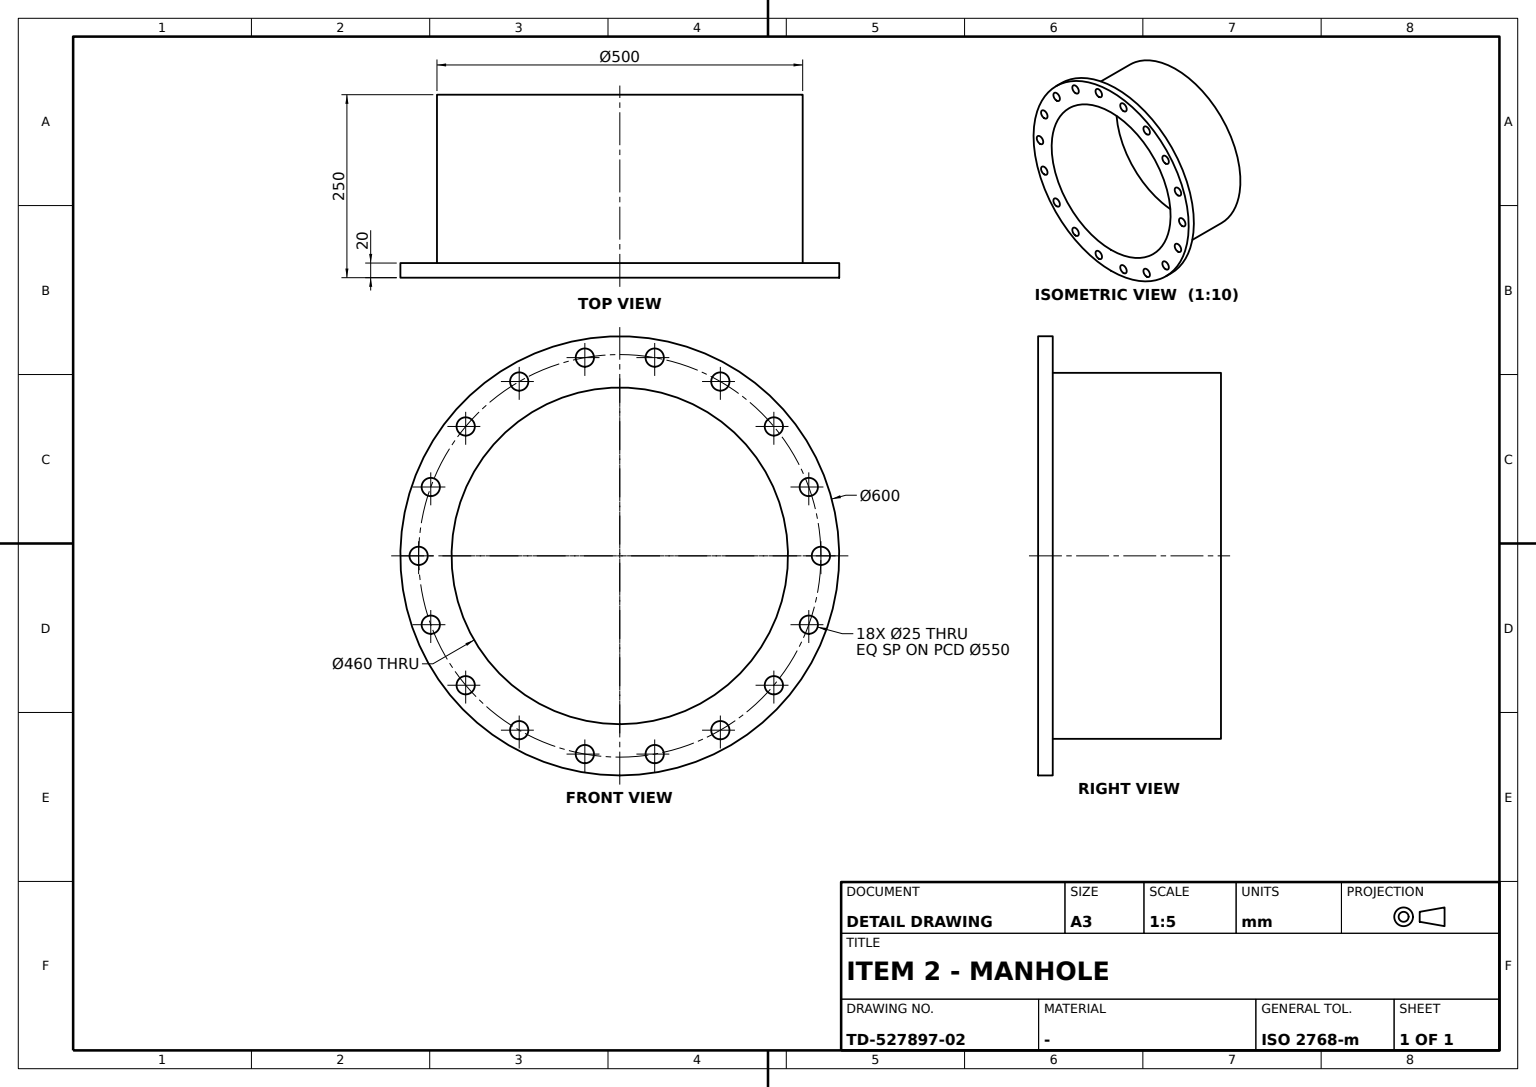
ISO-10303-21;
HEADER;
FILE_DESCRIPTION((''),'2;1');
FILE_NAME('','',(''),(''),'','','');
FILE_SCHEMA(('AUTOMOTIVE_DESIGN'));
ENDSEC;
DATA;
#1=APPLICATION_CONTEXT('');
#2=PRODUCT_CONTEXT('',#1,'mechanical');
#3=PRODUCT('','','',(#2));
#4=PRODUCT_DEFINITION_FORMATION('','',#3);
#5=PRODUCT_DEFINITION_CONTEXT('',#1,'design');
#6=PRODUCT_DEFINITION('','',#4,#5);
#7=PRODUCT_DEFINITION_SHAPE('','',#6);
#8=(LENGTH_UNIT()NAMED_UNIT(*)SI_UNIT(.MILLI.,.METRE.));
#9=(NAMED_UNIT(*)PLANE_ANGLE_UNIT()SI_UNIT($,.RADIAN.));
#10=(NAMED_UNIT(*)SI_UNIT($,.STERADIAN.)SOLID_ANGLE_UNIT());
#11=UNCERTAINTY_MEASURE_WITH_UNIT(LENGTH_MEASURE(0.005),#8,'distance_accuracy_value','');
#12=(GEOMETRIC_REPRESENTATION_CONTEXT(3)GLOBAL_UNCERTAINTY_ASSIGNED_CONTEXT((#11))GLOBAL_UNIT_ASSIGNED_CONTEXT((#8,#9,#10))REPRESENTATION_CONTEXT('',''));
#13=CARTESIAN_POINT('',(250.656986,-137.5,2750.));
#14=VERTEX_POINT('',#13);
#15=CARTESIAN_POINT('',(238.156986,-137.5,2750.));
#16=DIRECTION('',(0.,0.,1.));
#17=DIRECTION('',(1.,0.,0.));
#18=AXIS2_PLACEMENT_3D('',#15,#16,#17);
#19=CIRCLE('',#18,12.5);
#20=EDGE_CURVE('',#14,#14,#19,.T.);
#21=ORIENTED_EDGE('',*,*,#20,.T.);
#22=EDGE_LOOP('',(#21));
#23=FACE_BOUND('',#22,.T.);
#24=CARTESIAN_POINT('',(250.656986,-137.5,2730.));
#25=VERTEX_POINT('',#24);
#26=CARTESIAN_POINT('',(238.156986,-137.5,2730.));
#27=AXIS2_PLACEMENT_3D('',#26,#16,#17);
#28=CIRCLE('',#27,12.5);
#29=EDGE_CURVE('',#25,#25,#28,.T.);
#30=ORIENTED_EDGE('',*,*,#29,.F.);
#31=EDGE_LOOP('',(#30));
#32=FACE_BOUND('',#31,.T.);
#33=CARTESIAN_POINT('',(238.156986,-137.5,2740.));
#34=AXIS2_PLACEMENT_3D('',#33,#16,#17);
#35=CYLINDRICAL_SURFACE('',#34,12.5);
#36=ADVANCED_FACE('',(#23,#32),#35,.F.);
#37=CARTESIAN_POINT('',(-164.266593,-210.662222,2750.));
#38=VERTEX_POINT('',#37);
#39=CARTESIAN_POINT('',(-176.766593,-210.662222,2750.));
#40=AXIS2_PLACEMENT_3D('',#39,#16,#17);
#41=CIRCLE('',#40,12.5);
#42=EDGE_CURVE('',#38,#38,#41,.T.);
#43=ORIENTED_EDGE('',*,*,#42,.T.);
#44=EDGE_LOOP('',(#43));
#45=FACE_BOUND('',#44,.T.);
#46=CARTESIAN_POINT('',(-164.266593,-210.662222,2730.));
#47=VERTEX_POINT('',#46);
#48=CARTESIAN_POINT('',(-176.766593,-210.662222,2730.));
#49=AXIS2_PLACEMENT_3D('',#48,#16,#17);
#50=CIRCLE('',#49,12.5);
#51=EDGE_CURVE('',#47,#47,#50,.T.);
#52=ORIENTED_EDGE('',*,*,#51,.F.);
#53=EDGE_LOOP('',(#52));
#54=FACE_BOUND('',#53,.T.);
#55=CARTESIAN_POINT('',(-176.766593,-210.662222,2740.));
#56=AXIS2_PLACEMENT_3D('',#55,#16,#17);
#57=CYLINDRICAL_SURFACE('',#56,12.5);
#58=ADVANCED_FACE('',(#45,#54),#57,.F.);
#59=CARTESIAN_POINT('',(-81.555539,258.415471,2730.));
#60=VERTEX_POINT('',#59);
#61=CARTESIAN_POINT('',(-94.055539,258.415471,2730.));
#62=AXIS2_PLACEMENT_3D('',#61,#16,#17);
#63=CIRCLE('',#62,12.5);
#64=EDGE_CURVE('',#60,#60,#63,.T.);
#65=ORIENTED_EDGE('',*,*,#64,.F.);
#66=EDGE_LOOP('',(#65));
#67=FACE_BOUND('',#66,.T.);
#68=CARTESIAN_POINT('',(-81.555539,258.415471,2750.));
#69=VERTEX_POINT('',#68);
#70=CARTESIAN_POINT('',(-94.055539,258.415471,2750.));
#71=AXIS2_PLACEMENT_3D('',#70,#16,#17);
#72=CIRCLE('',#71,12.5);
#73=EDGE_CURVE('',#69,#69,#72,.T.);
#74=ORIENTED_EDGE('',*,*,#73,.T.);
#75=EDGE_LOOP('',(#74));
#76=FACE_BOUND('',#75,.T.);
#77=CARTESIAN_POINT('',(-94.055539,258.415471,2740.));
#78=AXIS2_PLACEMENT_3D('',#77,#16,#17);
#79=CYLINDRICAL_SURFACE('',#78,12.5);
#80=ADVANCED_FACE('',(#67,#76),#79,.F.);
#81=CARTESIAN_POINT('',(230.,0.,2750.));
#82=VERTEX_POINT('',#81);
#83=CARTESIAN_POINT('',(0.,0.,2750.));
#84=AXIS2_PLACEMENT_3D('',#83,#16,#17);
#85=CIRCLE('',#84,230.);
#86=EDGE_CURVE('',#82,#82,#85,.T.);
#87=ORIENTED_EDGE('',*,*,#86,.T.);
#88=EDGE_LOOP('',(#87));
#89=FACE_BOUND('',#88,.T.);
#90=CARTESIAN_POINT('',(230.,0.,2500.));
#91=VERTEX_POINT('',#90);
#92=CARTESIAN_POINT('',(0.,0.,2500.));
#93=AXIS2_PLACEMENT_3D('',#92,#16,#17);
#94=CIRCLE('',#93,230.);
#95=EDGE_CURVE('',#91,#91,#94,.T.);
#96=ORIENTED_EDGE('',*,*,#95,.F.);
#97=EDGE_LOOP('',(#96));
#98=FACE_BOUND('',#97,.T.);
#99=CARTESIAN_POINT('',(0.,0.,2625.));
#100=AXIS2_PLACEMENT_3D('',#99,#16,#17);
#101=CYLINDRICAL_SURFACE('',#100,230.);
#102=ADVANCED_FACE('',(#89,#98),#101,.F.);
#103=CARTESIAN_POINT('',(-225.656986,137.5,2730.));
#104=VERTEX_POINT('',#103);
#105=CARTESIAN_POINT('',(-238.156986,137.5,2730.));
#106=AXIS2_PLACEMENT_3D('',#105,#16,#17);
#107=CIRCLE('',#106,12.5);
#108=EDGE_CURVE('',#104,#104,#107,.T.);
#109=ORIENTED_EDGE('',*,*,#108,.F.);
#110=EDGE_LOOP('',(#109));
#111=FACE_BOUND('',#110,.T.);
#112=CARTESIAN_POINT('',(-225.656986,137.5,2750.));
#113=VERTEX_POINT('',#112);
#114=CARTESIAN_POINT('',(-238.156986,137.5,2750.));
#115=AXIS2_PLACEMENT_3D('',#114,#16,#17);
#116=CIRCLE('',#115,12.5);
#117=EDGE_CURVE('',#113,#113,#116,.T.);
#118=ORIENTED_EDGE('',*,*,#117,.T.);
#119=EDGE_LOOP('',(#118));
#120=FACE_BOUND('',#119,.T.);
#121=CARTESIAN_POINT('',(-238.156986,137.5,2740.));
#122=AXIS2_PLACEMENT_3D('',#121,#16,#17);
#123=CYLINDRICAL_SURFACE('',#122,12.5);
#124=ADVANCED_FACE('',(#111,#120),#123,.F.);
#125=CARTESIAN_POINT('',(250.,0.,2500.));
#126=VERTEX_POINT('',#125);
#127=CIRCLE('',#93,250.);
#128=EDGE_CURVE('',#126,#126,#127,.T.);
#129=ORIENTED_EDGE('',*,*,#128,.F.);
#130=EDGE_LOOP('',(#129));
#131=FACE_BOUND('',#130,.T.);
#132=ORIENTED_EDGE('',*,*,#95,.T.);
#133=EDGE_LOOP('',(#132));
#134=FACE_BOUND('',#133,.T.);
#135=PLANE('',#93);
#136=ADVANCED_FACE('',(#131,#134),#135,.F.);
#137=CARTESIAN_POINT('',(12.5,275.,2750.));
#138=VERTEX_POINT('',#137);
#139=CARTESIAN_POINT('',(0.,275.,2750.));
#140=AXIS2_PLACEMENT_3D('',#139,#16,#17);
#141=CIRCLE('',#140,12.5);
#142=EDGE_CURVE('',#138,#138,#141,.T.);
#143=ORIENTED_EDGE('',*,*,#142,.T.);
#144=EDGE_LOOP('',(#143));
#145=FACE_BOUND('',#144,.T.);
#146=CARTESIAN_POINT('',(12.5,275.,2730.));
#147=VERTEX_POINT('',#146);
#148=CARTESIAN_POINT('',(0.,275.,2730.));
#149=AXIS2_PLACEMENT_3D('',#148,#16,#17);
#150=CIRCLE('',#149,12.5);
#151=EDGE_CURVE('',#147,#147,#150,.T.);
#152=ORIENTED_EDGE('',*,*,#151,.F.);
#153=EDGE_LOOP('',(#152));
#154=FACE_BOUND('',#153,.T.);
#155=CARTESIAN_POINT('',(0.,275.,2740.));
#156=AXIS2_PLACEMENT_3D('',#155,#16,#17);
#157=CYLINDRICAL_SURFACE('',#156,12.5);
#158=ADVANCED_FACE('',(#145,#154),#157,.F.);
#159=CARTESIAN_POINT('',(250.,0.,2730.));
#160=VERTEX_POINT('',#159);
#161=CARTESIAN_POINT('',(0.,0.,2730.));
#162=AXIS2_PLACEMENT_3D('',#161,#16,#17);
#163=CIRCLE('',#162,250.);
#164=EDGE_CURVE('',#160,#160,#163,.T.);
#165=ORIENTED_EDGE('',*,*,#164,.F.);
#166=EDGE_LOOP('',(#165));
#167=FACE_BOUND('',#166,.T.);
#168=ORIENTED_EDGE('',*,*,#128,.T.);
#169=EDGE_LOOP('',(#168));
#170=FACE_BOUND('',#169,.T.);
#171=CARTESIAN_POINT('',(0.,0.,2740.));
#172=AXIS2_PLACEMENT_3D('',#171,#16,#17);
#173=CYLINDRICAL_SURFACE('',#172,250.);
#174=ADVANCED_FACE('',(#167,#170),#173,.T.);
#175=CARTESIAN_POINT('',(-164.266593,210.662222,2750.));
#176=VERTEX_POINT('',#175);
#177=CARTESIAN_POINT('',(-176.766593,210.662222,2750.));
#178=AXIS2_PLACEMENT_3D('',#177,#16,#17);
#179=CIRCLE('',#178,12.5);
#180=EDGE_CURVE('',#176,#176,#179,.T.);
#181=ORIENTED_EDGE('',*,*,#180,.T.);
#182=EDGE_LOOP('',(#181));
#183=FACE_BOUND('',#182,.T.);
#184=CARTESIAN_POINT('',(-164.266593,210.662222,2730.));
#185=VERTEX_POINT('',#184);
#186=CARTESIAN_POINT('',(-176.766593,210.662222,2730.));
#187=AXIS2_PLACEMENT_3D('',#186,#16,#17);
#188=CIRCLE('',#187,12.5);
#189=EDGE_CURVE('',#185,#185,#188,.T.);
#190=ORIENTED_EDGE('',*,*,#189,.F.);
#191=EDGE_LOOP('',(#190));
#192=FACE_BOUND('',#191,.T.);
#193=CARTESIAN_POINT('',(-176.766593,210.662222,2740.));
#194=AXIS2_PLACEMENT_3D('',#193,#16,#17);
#195=CYLINDRICAL_SURFACE('',#194,12.5);
#196=ADVANCED_FACE('',(#183,#192),#195,.F.);
#197=CARTESIAN_POINT('',(283.322132,-47.753249,2730.));
#198=VERTEX_POINT('',#197);
#199=CARTESIAN_POINT('',(270.822132,-47.753249,2730.));
#200=AXIS2_PLACEMENT_3D('',#199,#16,#17);
#201=CIRCLE('',#200,12.5);
#202=EDGE_CURVE('',#198,#198,#201,.T.);
#203=ORIENTED_EDGE('',*,*,#202,.F.);
#204=EDGE_LOOP('',(#203));
#205=FACE_BOUND('',#204,.T.);
#206=CARTESIAN_POINT('',(283.322132,-47.753249,2750.));
#207=VERTEX_POINT('',#206);
#208=CARTESIAN_POINT('',(270.822132,-47.753249,2750.));
#209=AXIS2_PLACEMENT_3D('',#208,#16,#17);
#210=CIRCLE('',#209,12.5);
#211=EDGE_CURVE('',#207,#207,#210,.T.);
#212=ORIENTED_EDGE('',*,*,#211,.T.);
#213=EDGE_LOOP('',(#212));
#214=FACE_BOUND('',#213,.T.);
#215=CARTESIAN_POINT('',(270.822132,-47.753249,2740.));
#216=AXIS2_PLACEMENT_3D('',#215,#16,#17);
#217=CYLINDRICAL_SURFACE('',#216,12.5);
#218=ADVANCED_FACE('',(#205,#214),#217,.F.);
#219=CARTESIAN_POINT('',(-225.656986,-137.5,2730.));
#220=VERTEX_POINT('',#219);
#221=CARTESIAN_POINT('',(-238.156986,-137.5,2730.));
#222=AXIS2_PLACEMENT_3D('',#221,#16,#17);
#223=CIRCLE('',#222,12.5);
#224=EDGE_CURVE('',#220,#220,#223,.T.);
#225=ORIENTED_EDGE('',*,*,#224,.F.);
#226=EDGE_LOOP('',(#225));
#227=FACE_BOUND('',#226,.T.);
#228=CARTESIAN_POINT('',(-225.656986,-137.5,2750.));
#229=VERTEX_POINT('',#228);
#230=CARTESIAN_POINT('',(-238.156986,-137.5,2750.));
#231=AXIS2_PLACEMENT_3D('',#230,#16,#17);
#232=CIRCLE('',#231,12.5);
#233=EDGE_CURVE('',#229,#229,#232,.T.);
#234=ORIENTED_EDGE('',*,*,#233,.T.);
#235=EDGE_LOOP('',(#234));
#236=FACE_BOUND('',#235,.T.);
#237=CARTESIAN_POINT('',(-238.156986,-137.5,2740.));
#238=AXIS2_PLACEMENT_3D('',#237,#16,#17);
#239=CYLINDRICAL_SURFACE('',#238,12.5);
#240=ADVANCED_FACE('',(#227,#236),#239,.F.);
#241=CARTESIAN_POINT('',(250.656986,137.5,2730.));
#242=VERTEX_POINT('',#241);
#243=CARTESIAN_POINT('',(238.156986,137.5,2730.));
#244=AXIS2_PLACEMENT_3D('',#243,#16,#17);
#245=CIRCLE('',#244,12.5);
#246=EDGE_CURVE('',#242,#242,#245,.T.);
#247=ORIENTED_EDGE('',*,*,#246,.F.);
#248=EDGE_LOOP('',(#247));
#249=FACE_BOUND('',#248,.T.);
#250=CARTESIAN_POINT('',(250.656986,137.5,2750.));
#251=VERTEX_POINT('',#250);
#252=CARTESIAN_POINT('',(238.156986,137.5,2750.));
#253=AXIS2_PLACEMENT_3D('',#252,#16,#17);
#254=CIRCLE('',#253,12.5);
#255=EDGE_CURVE('',#251,#251,#254,.T.);
#256=ORIENTED_EDGE('',*,*,#255,.T.);
#257=EDGE_LOOP('',(#256));
#258=FACE_BOUND('',#257,.T.);
#259=CARTESIAN_POINT('',(238.156986,137.5,2740.));
#260=AXIS2_PLACEMENT_3D('',#259,#16,#17);
#261=CYLINDRICAL_SURFACE('',#260,12.5);
#262=ADVANCED_FACE('',(#249,#258),#261,.F.);
#263=CARTESIAN_POINT('',(-81.555539,-258.415471,2750.));
#264=VERTEX_POINT('',#263);
#265=CARTESIAN_POINT('',(-94.055539,-258.415471,2750.));
#266=AXIS2_PLACEMENT_3D('',#265,#16,#17);
#267=CIRCLE('',#266,12.5);
#268=EDGE_CURVE('',#264,#264,#267,.T.);
#269=ORIENTED_EDGE('',*,*,#268,.T.);
#270=EDGE_LOOP('',(#269));
#271=FACE_BOUND('',#270,.T.);
#272=CARTESIAN_POINT('',(-81.555539,-258.415471,2730.));
#273=VERTEX_POINT('',#272);
#274=CARTESIAN_POINT('',(-94.055539,-258.415471,2730.));
#275=AXIS2_PLACEMENT_3D('',#274,#16,#17);
#276=CIRCLE('',#275,12.5);
#277=EDGE_CURVE('',#273,#273,#276,.T.);
#278=ORIENTED_EDGE('',*,*,#277,.F.);
#279=EDGE_LOOP('',(#278));
#280=FACE_BOUND('',#279,.T.);
#281=CARTESIAN_POINT('',(-94.055539,-258.415471,2740.));
#282=AXIS2_PLACEMENT_3D('',#281,#16,#17);
#283=CYLINDRICAL_SURFACE('',#282,12.5);
#284=ADVANCED_FACE('',(#271,#280),#283,.F.);
#285=ORIENTED_EDGE('',*,*,#180,.F.);
#286=EDGE_LOOP('',(#285));
#287=FACE_BOUND('',#286,.T.);
#288=CARTESIAN_POINT('',(283.322132,47.753249,2750.));
#289=VERTEX_POINT('',#288);
#290=CARTESIAN_POINT('',(270.822132,47.753249,2750.));
#291=AXIS2_PLACEMENT_3D('',#290,#16,#17);
#292=CIRCLE('',#291,12.5);
#293=EDGE_CURVE('',#289,#289,#292,.T.);
#294=ORIENTED_EDGE('',*,*,#293,.F.);
#295=EDGE_LOOP('',(#294));
#296=FACE_BOUND('',#295,.T.);
#297=ORIENTED_EDGE('',*,*,#20,.F.);
#298=EDGE_LOOP('',(#297));
#299=FACE_BOUND('',#298,.T.);
#300=CARTESIAN_POINT('',(189.266593,-210.662222,2750.));
#301=VERTEX_POINT('',#300);
#302=CARTESIAN_POINT('',(176.766593,-210.662222,2750.));
#303=AXIS2_PLACEMENT_3D('',#302,#16,#17);
#304=CIRCLE('',#303,12.5);
#305=EDGE_CURVE('',#301,#301,#304,.T.);
#306=ORIENTED_EDGE('',*,*,#305,.F.);
#307=EDGE_LOOP('',(#306));
#308=FACE_BOUND('',#307,.T.);
#309=CARTESIAN_POINT('',(189.266593,210.662222,2750.));
#310=VERTEX_POINT('',#309);
#311=CARTESIAN_POINT('',(176.766593,210.662222,2750.));
#312=AXIS2_PLACEMENT_3D('',#311,#16,#17);
#313=CIRCLE('',#312,12.5);
#314=EDGE_CURVE('',#310,#310,#313,.T.);
#315=ORIENTED_EDGE('',*,*,#314,.F.);
#316=EDGE_LOOP('',(#315));
#317=FACE_BOUND('',#316,.T.);
#318=ORIENTED_EDGE('',*,*,#255,.F.);
#319=EDGE_LOOP('',(#318));
#320=FACE_BOUND('',#319,.T.);
#321=CARTESIAN_POINT('',(12.5,-275.,2750.));
#322=VERTEX_POINT('',#321);
#323=CARTESIAN_POINT('',(0.,-275.,2750.));
#324=AXIS2_PLACEMENT_3D('',#323,#16,#17);
#325=CIRCLE('',#324,12.5);
#326=EDGE_CURVE('',#322,#322,#325,.T.);
#327=ORIENTED_EDGE('',*,*,#326,.F.);
#328=EDGE_LOOP('',(#327));
#329=FACE_BOUND('',#328,.T.);
#330=ORIENTED_EDGE('',*,*,#86,.F.);
#331=EDGE_LOOP('',(#330));
#332=FACE_BOUND('',#331,.T.);
#333=ORIENTED_EDGE('',*,*,#233,.F.);
#334=EDGE_LOOP('',(#333));
#335=FACE_BOUND('',#334,.T.);
#336=CARTESIAN_POINT('',(-258.322132,47.753249,2750.));
#337=VERTEX_POINT('',#336);
#338=CARTESIAN_POINT('',(-270.822132,47.753249,2750.));
#339=AXIS2_PLACEMENT_3D('',#338,#16,#17);
#340=CIRCLE('',#339,12.5);
#341=EDGE_CURVE('',#337,#337,#340,.T.);
#342=ORIENTED_EDGE('',*,*,#341,.F.);
#343=EDGE_LOOP('',(#342));
#344=FACE_BOUND('',#343,.T.);
#345=ORIENTED_EDGE('',*,*,#73,.F.);
#346=EDGE_LOOP('',(#345));
#347=FACE_BOUND('',#346,.T.);
#348=ORIENTED_EDGE('',*,*,#211,.F.);
#349=EDGE_LOOP('',(#348));
#350=FACE_BOUND('',#349,.T.);
#351=CARTESIAN_POINT('',(-258.322132,-47.753249,2750.));
#352=VERTEX_POINT('',#351);
#353=CARTESIAN_POINT('',(-270.822132,-47.753249,2750.));
#354=AXIS2_PLACEMENT_3D('',#353,#16,#17);
#355=CIRCLE('',#354,12.5);
#356=EDGE_CURVE('',#352,#352,#355,.T.);
#357=ORIENTED_EDGE('',*,*,#356,.F.);
#358=EDGE_LOOP('',(#357));
#359=FACE_BOUND('',#358,.T.);
#360=ORIENTED_EDGE('',*,*,#117,.F.);
#361=EDGE_LOOP('',(#360));
#362=FACE_BOUND('',#361,.T.);
#363=ORIENTED_EDGE('',*,*,#268,.F.);
#364=EDGE_LOOP('',(#363));
#365=FACE_BOUND('',#364,.T.);
#366=ORIENTED_EDGE('',*,*,#42,.F.);
#367=EDGE_LOOP('',(#366));
#368=FACE_BOUND('',#367,.T.);
#369=CARTESIAN_POINT('',(106.555539,258.415471,2750.));
#370=VERTEX_POINT('',#369);
#371=CARTESIAN_POINT('',(94.055539,258.415471,2750.));
#372=AXIS2_PLACEMENT_3D('',#371,#16,#17);
#373=CIRCLE('',#372,12.5);
#374=EDGE_CURVE('',#370,#370,#373,.T.);
#375=ORIENTED_EDGE('',*,*,#374,.F.);
#376=EDGE_LOOP('',(#375));
#377=FACE_BOUND('',#376,.T.);
#378=CARTESIAN_POINT('',(300.,0.,2750.));
#379=VERTEX_POINT('',#378);
#380=CIRCLE('',#84,300.);
#381=EDGE_CURVE('',#379,#379,#380,.T.);
#382=ORIENTED_EDGE('',*,*,#381,.T.);
#383=EDGE_LOOP('',(#382));
#384=FACE_BOUND('',#383,.T.);
#385=CARTESIAN_POINT('',(106.555539,-258.415471,2750.));
#386=VERTEX_POINT('',#385);
#387=CARTESIAN_POINT('',(94.055539,-258.415471,2750.));
#388=AXIS2_PLACEMENT_3D('',#387,#16,#17);
#389=CIRCLE('',#388,12.5);
#390=EDGE_CURVE('',#386,#386,#389,.T.);
#391=ORIENTED_EDGE('',*,*,#390,.F.);
#392=EDGE_LOOP('',(#391));
#393=FACE_BOUND('',#392,.T.);
#394=ORIENTED_EDGE('',*,*,#142,.F.);
#395=EDGE_LOOP('',(#394));
#396=FACE_BOUND('',#395,.T.);
#397=PLANE('',#84);
#398=ADVANCED_FACE('',(#287,#296,#299,#308,#317,#320,#329,#332,#335,#344,#347,#350,#359,#362,#365,#368,#377,#384,#393,#396),#397,.T.);
#399=ORIENTED_EDGE('',*,*,#381,.F.);
#400=EDGE_LOOP('',(#399));
#401=FACE_BOUND('',#400,.T.);
#402=CARTESIAN_POINT('',(300.,0.,2730.));
#403=VERTEX_POINT('',#402);
#404=CIRCLE('',#162,300.);
#405=EDGE_CURVE('',#403,#403,#404,.T.);
#406=ORIENTED_EDGE('',*,*,#405,.T.);
#407=EDGE_LOOP('',(#406));
#408=FACE_BOUND('',#407,.T.);
#409=CYLINDRICAL_SURFACE('',#172,300.);
#410=ADVANCED_FACE('',(#401,#408),#409,.T.);
#411=CARTESIAN_POINT('',(283.322132,47.753249,2730.));
#412=VERTEX_POINT('',#411);
#413=CARTESIAN_POINT('',(270.822132,47.753249,2730.));
#414=AXIS2_PLACEMENT_3D('',#413,#16,#17);
#415=CIRCLE('',#414,12.5);
#416=EDGE_CURVE('',#412,#412,#415,.T.);
#417=ORIENTED_EDGE('',*,*,#416,.F.);
#418=EDGE_LOOP('',(#417));
#419=FACE_BOUND('',#418,.T.);
#420=ORIENTED_EDGE('',*,*,#293,.T.);
#421=EDGE_LOOP('',(#420));
#422=FACE_BOUND('',#421,.T.);
#423=CARTESIAN_POINT('',(270.822132,47.753249,2740.));
#424=AXIS2_PLACEMENT_3D('',#423,#16,#17);
#425=CYLINDRICAL_SURFACE('',#424,12.5);
#426=ADVANCED_FACE('',(#419,#422),#425,.F.);
#427=CARTESIAN_POINT('',(-258.322132,47.753249,2730.));
#428=VERTEX_POINT('',#427);
#429=CARTESIAN_POINT('',(-270.822132,47.753249,2730.));
#430=AXIS2_PLACEMENT_3D('',#429,#16,#17);
#431=CIRCLE('',#430,12.5);
#432=EDGE_CURVE('',#428,#428,#431,.T.);
#433=ORIENTED_EDGE('',*,*,#432,.F.);
#434=EDGE_LOOP('',(#433));
#435=FACE_BOUND('',#434,.T.);
#436=ORIENTED_EDGE('',*,*,#341,.T.);
#437=EDGE_LOOP('',(#436));
#438=FACE_BOUND('',#437,.T.);
#439=CARTESIAN_POINT('',(-270.822132,47.753249,2740.));
#440=AXIS2_PLACEMENT_3D('',#439,#16,#17);
#441=CYLINDRICAL_SURFACE('',#440,12.5);
#442=ADVANCED_FACE('',(#435,#438),#441,.F.);
#443=CARTESIAN_POINT('',(189.266593,-210.662222,2730.));
#444=VERTEX_POINT('',#443);
#445=CARTESIAN_POINT('',(176.766593,-210.662222,2730.));
#446=AXIS2_PLACEMENT_3D('',#445,#16,#17);
#447=CIRCLE('',#446,12.5);
#448=EDGE_CURVE('',#444,#444,#447,.T.);
#449=ORIENTED_EDGE('',*,*,#448,.F.);
#450=EDGE_LOOP('',(#449));
#451=FACE_BOUND('',#450,.T.);
#452=ORIENTED_EDGE('',*,*,#305,.T.);
#453=EDGE_LOOP('',(#452));
#454=FACE_BOUND('',#453,.T.);
#455=CARTESIAN_POINT('',(176.766593,-210.662222,2740.));
#456=AXIS2_PLACEMENT_3D('',#455,#16,#17);
#457=CYLINDRICAL_SURFACE('',#456,12.5);
#458=ADVANCED_FACE('',(#451,#454),#457,.F.);
#459=ORIENTED_EDGE('',*,*,#374,.T.);
#460=EDGE_LOOP('',(#459));
#461=FACE_BOUND('',#460,.T.);
#462=CARTESIAN_POINT('',(106.555539,258.415471,2730.));
#463=VERTEX_POINT('',#462);
#464=CARTESIAN_POINT('',(94.055539,258.415471,2730.));
#465=AXIS2_PLACEMENT_3D('',#464,#16,#17);
#466=CIRCLE('',#465,12.5);
#467=EDGE_CURVE('',#463,#463,#466,.T.);
#468=ORIENTED_EDGE('',*,*,#467,.F.);
#469=EDGE_LOOP('',(#468));
#470=FACE_BOUND('',#469,.T.);
#471=CARTESIAN_POINT('',(94.055539,258.415471,2740.));
#472=AXIS2_PLACEMENT_3D('',#471,#16,#17);
#473=CYLINDRICAL_SURFACE('',#472,12.5);
#474=ADVANCED_FACE('',(#461,#470),#473,.F.);
#475=CARTESIAN_POINT('',(106.555539,-258.415471,2730.));
#476=VERTEX_POINT('',#475);
#477=CARTESIAN_POINT('',(94.055539,-258.415471,2730.));
#478=AXIS2_PLACEMENT_3D('',#477,#16,#17);
#479=CIRCLE('',#478,12.5);
#480=EDGE_CURVE('',#476,#476,#479,.T.);
#481=ORIENTED_EDGE('',*,*,#480,.F.);
#482=EDGE_LOOP('',(#481));
#483=FACE_BOUND('',#482,.T.);
#484=ORIENTED_EDGE('',*,*,#390,.T.);
#485=EDGE_LOOP('',(#484));
#486=FACE_BOUND('',#485,.T.);
#487=CARTESIAN_POINT('',(94.055539,-258.415471,2740.));
#488=AXIS2_PLACEMENT_3D('',#487,#16,#17);
#489=CYLINDRICAL_SURFACE('',#488,12.5);
#490=ADVANCED_FACE('',(#483,#486),#489,.F.);
#491=ORIENTED_EDGE('',*,*,#356,.T.);
#492=EDGE_LOOP('',(#491));
#493=FACE_BOUND('',#492,.T.);
#494=CARTESIAN_POINT('',(-258.322132,-47.753249,2730.));
#495=VERTEX_POINT('',#494);
#496=CARTESIAN_POINT('',(-270.822132,-47.753249,2730.));
#497=AXIS2_PLACEMENT_3D('',#496,#16,#17);
#498=CIRCLE('',#497,12.5);
#499=EDGE_CURVE('',#495,#495,#498,.T.);
#500=ORIENTED_EDGE('',*,*,#499,.F.);
#501=EDGE_LOOP('',(#500));
#502=FACE_BOUND('',#501,.T.);
#503=CARTESIAN_POINT('',(-270.822132,-47.753249,2740.));
#504=AXIS2_PLACEMENT_3D('',#503,#16,#17);
#505=CYLINDRICAL_SURFACE('',#504,12.5);
#506=ADVANCED_FACE('',(#493,#502),#505,.F.);
#507=CARTESIAN_POINT('',(12.5,-275.,2730.));
#508=VERTEX_POINT('',#507);
#509=CARTESIAN_POINT('',(0.,-275.,2730.));
#510=AXIS2_PLACEMENT_3D('',#509,#16,#17);
#511=CIRCLE('',#510,12.5);
#512=EDGE_CURVE('',#508,#508,#511,.T.);
#513=ORIENTED_EDGE('',*,*,#512,.F.);
#514=EDGE_LOOP('',(#513));
#515=FACE_BOUND('',#514,.T.);
#516=ORIENTED_EDGE('',*,*,#326,.T.);
#517=EDGE_LOOP('',(#516));
#518=FACE_BOUND('',#517,.T.);
#519=CARTESIAN_POINT('',(0.,-275.,2740.));
#520=AXIS2_PLACEMENT_3D('',#519,#16,#17);
#521=CYLINDRICAL_SURFACE('',#520,12.5);
#522=ADVANCED_FACE('',(#515,#518),#521,.F.);
#523=CARTESIAN_POINT('',(189.266593,210.662222,2730.));
#524=VERTEX_POINT('',#523);
#525=CARTESIAN_POINT('',(176.766593,210.662222,2730.));
#526=AXIS2_PLACEMENT_3D('',#525,#16,#17);
#527=CIRCLE('',#526,12.5);
#528=EDGE_CURVE('',#524,#524,#527,.T.);
#529=ORIENTED_EDGE('',*,*,#528,.F.);
#530=EDGE_LOOP('',(#529));
#531=FACE_BOUND('',#530,.T.);
#532=ORIENTED_EDGE('',*,*,#314,.T.);
#533=EDGE_LOOP('',(#532));
#534=FACE_BOUND('',#533,.T.);
#535=CARTESIAN_POINT('',(176.766593,210.662222,2740.));
#536=AXIS2_PLACEMENT_3D('',#535,#16,#17);
#537=CYLINDRICAL_SURFACE('',#536,12.5);
#538=ADVANCED_FACE('',(#531,#534),#537,.F.);
#539=ORIENTED_EDGE('',*,*,#467,.T.);
#540=EDGE_LOOP('',(#539));
#541=FACE_BOUND('',#540,.T.);
#542=ORIENTED_EDGE('',*,*,#512,.T.);
#543=EDGE_LOOP('',(#542));
#544=FACE_BOUND('',#543,.T.);
#545=ORIENTED_EDGE('',*,*,#448,.T.);
#546=EDGE_LOOP('',(#545));
#547=FACE_BOUND('',#546,.T.);
#548=ORIENTED_EDGE('',*,*,#416,.T.);
#549=EDGE_LOOP('',(#548));
#550=FACE_BOUND('',#549,.T.);
#551=ORIENTED_EDGE('',*,*,#277,.T.);
#552=EDGE_LOOP('',(#551));
#553=FACE_BOUND('',#552,.T.);
#554=ORIENTED_EDGE('',*,*,#224,.T.);
#555=EDGE_LOOP('',(#554));
#556=FACE_BOUND('',#555,.T.);
#557=ORIENTED_EDGE('',*,*,#528,.T.);
#558=EDGE_LOOP('',(#557));
#559=FACE_BOUND('',#558,.T.);
#560=ORIENTED_EDGE('',*,*,#151,.T.);
#561=EDGE_LOOP('',(#560));
#562=FACE_BOUND('',#561,.T.);
#563=ORIENTED_EDGE('',*,*,#246,.T.);
#564=EDGE_LOOP('',(#563));
#565=FACE_BOUND('',#564,.T.);
#566=ORIENTED_EDGE('',*,*,#432,.T.);
#567=EDGE_LOOP('',(#566));
#568=FACE_BOUND('',#567,.T.);
#569=ORIENTED_EDGE('',*,*,#189,.T.);
#570=EDGE_LOOP('',(#569));
#571=FACE_BOUND('',#570,.T.);
#572=ORIENTED_EDGE('',*,*,#405,.F.);
#573=EDGE_LOOP('',(#572));
#574=FACE_BOUND('',#573,.T.);
#575=ORIENTED_EDGE('',*,*,#164,.T.);
#576=EDGE_LOOP('',(#575));
#577=FACE_BOUND('',#576,.T.);
#578=ORIENTED_EDGE('',*,*,#202,.T.);
#579=EDGE_LOOP('',(#578));
#580=FACE_BOUND('',#579,.T.);
#581=ORIENTED_EDGE('',*,*,#64,.T.);
#582=EDGE_LOOP('',(#581));
#583=FACE_BOUND('',#582,.T.);
#584=ORIENTED_EDGE('',*,*,#480,.T.);
#585=EDGE_LOOP('',(#584));
#586=FACE_BOUND('',#585,.T.);
#587=ORIENTED_EDGE('',*,*,#108,.T.);
#588=EDGE_LOOP('',(#587));
#589=FACE_BOUND('',#588,.T.);
#590=ORIENTED_EDGE('',*,*,#29,.T.);
#591=EDGE_LOOP('',(#590));
#592=FACE_BOUND('',#591,.T.);
#593=ORIENTED_EDGE('',*,*,#51,.T.);
#594=EDGE_LOOP('',(#593));
#595=FACE_BOUND('',#594,.T.);
#596=ORIENTED_EDGE('',*,*,#499,.T.);
#597=EDGE_LOOP('',(#596));
#598=FACE_BOUND('',#597,.T.);
#599=PLANE('',#162);
#600=ADVANCED_FACE('',(#541,#544,#547,#550,#553,#556,#559,#562,#565,#568,#571,#574,#577,#580,#583,#586,#589,#592,#595,#598),#599,.F.);
#601=CLOSED_SHELL('',(#36,#58,#80,#102,#124,#136,#158,#174,#196,#218,#240,#262,#284,#398,#410,#426,#442,#458,#474,#490,#506,#522,#538,#600));
#602=MANIFOLD_SOLID_BREP('',#601);
#603=ADVANCED_BREP_SHAPE_REPRESENTATION('',(#602),#12);
#604=SHAPE_DEFINITION_REPRESENTATION(#7,#603);
ENDSEC;
END-ISO-10303-21;
